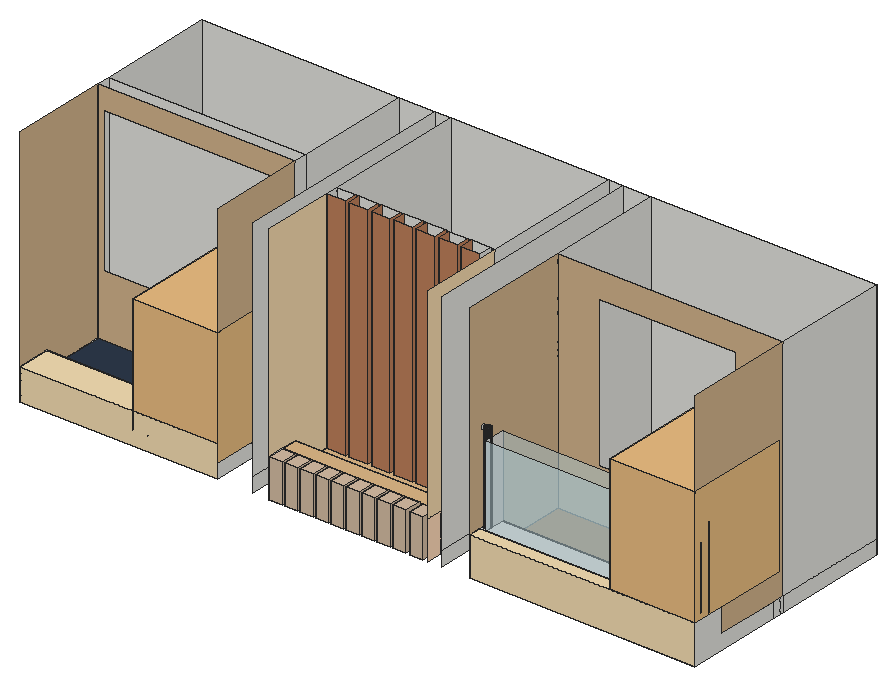
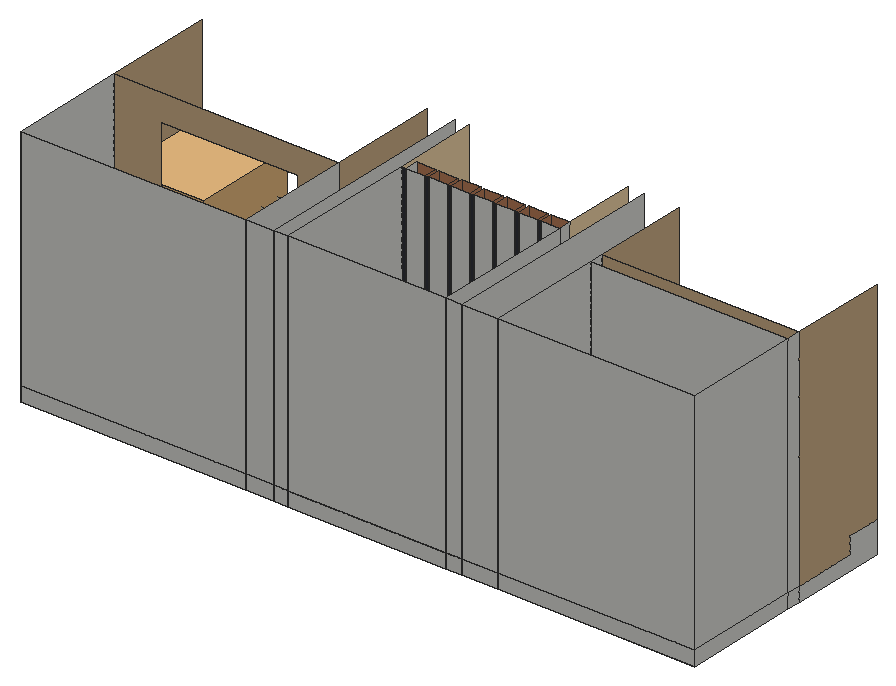
# SketchUp Ruby script. Lengths in inches.
U = 1.inch
M = Sketchup.active_model
def pt(a) = Geom::Point3d.new(a.map { |v| v * U })
def face(e, loops, mat)
  f = e.add_face(loops[0].map { |a| pt(a) })
  loops[1..].each { |l| e.add_face(l.map { |a| pt(a) }).erase! }
  f.material = f.back_material = mat if mat
  f
end
# faces: each face lists its corners as indices into pts; further lists are holes
def faces(e, pts, list, mat = nil) = list.each { |f| face(e, (f[0].is_a?(Array) ? f : [f]).map { |l| l.map { |i| pts[i] } }, mat) }
# xy, xz, yz: faces in a plane at the given z, y or x. An outline is a flat list of corners, or four numbers for a rectangle; further outlines are holes
def ring(l) = l.size == 4 ? [[l[0], l[1]], [l[2], l[1]], [l[2], l[3]], [l[0], l[3]]] : l.each_slice(2).to_a
def flat(e, list, mat, &to3) = list.each { |f| face(e, (f[0].is_a?(Array) ? f : [f]).map { |l| ring(l).map { |u, v| to3.(u, v) } }, mat) }
def xy(e, z, list, mat = nil) = flat(e, list, mat) { |x, y| [x, y, z] }
def xz(e, y, list, mat = nil) = flat(e, list, mat) { |x, z| [x, y, z] }
def yz(e, x, list, mat = nil) = flat(e, list, mat) { |y, z| [x, y, z] }
def lines(e, pts, list) = list.each { |a, b| e.add_line(pt(pts[a]), pt(pts[b])) }
# prism: a flat outline (further loops are holes) pulled along v
def prism(e, loops, v, mat = nil)
  f = face(e, loops, mat); d = Geom::Vector3d.new(v.map { |x| x * U })
  f.pushpull(f.normal.samedirection?(d) ? d.length : -d.length)
end
def box(e, o, s, mat = nil) = prism(e, [[o, [o[0] + s[0], o[1], o[2]], [o[0] + s[0], o[1] + s[1], o[2]], [o[0], o[1] + s[1], o[2]]]], [0, 0, s[2]], mat)
def at(x, y, z, deg = 0) = Geom::Transformation.translation(pt([x, y, z])) * Geom::Transformation.rotation(ORIGIN, Z_AXIS, deg.degrees)
def axes(o, x, y, z) = Geom::Transformation.new([*x, 0, *y, 0, *z, 0, *pt(o).to_a, 1])
def part(name) = M.definitions.add(name)
# library, detail: a bought-in or finely detailed component or shape, given as its bounding box
def library(name, o, s) = part(name).tap { |d| box(d.entities, o, s) }
def detail(e, o, s) = box(e.add_group.entities, o, s)
def put(e, d, t, mat = nil) = e.add_instance(d, t).tap { |i| i.material = mat if mat }
def group(e, t, mat = nil) = e.add_group.tap { |g| g.transformation = t; g.material = mat if mat }.entities
root = M.entities
M.materials.add("[0027_PeachPuff]").color = [255, 218, 185]
M.materials.add("[0034_Wheat]").color = [245, 222, 179]
M.materials.add("[0035_Tan]").color = [210, 180, 140]
M.materials.add("[0036_BurlyWood]1").color = [222, 184, 135]
M.materials.add("[Formica Beige]").color = [247, 219, 174]
M.materials.add("[Formica Laminate Dark]").color = [50, 53, 60]
M.materials.add("[Formica Laminate Light]").color = [213, 189, 164]
M.materials.add("[Leather Blue]").color = [45, 57, 74]
M.materials.add("[Translucent Glass Safety]").color = [204, 235, 244]
M.materials["[Translucent Glass Safety]"].alpha = 0.5
M.materials.add("[Wood Square Tile 02]").color = [160, 95, 34]
M.materials.add("[Wood Veneer 02]").color = [190, 128, 91]
c1 = library("chau cay",[-24.34,-109.24,0],[56.46,62.58,79.69])
xy(root,3076.3125,[[800.41,467.67,800.41,584.29,1272.8,584.29,1272.8,467.67,1233.94,467.67,1233.94,495.54,1224.82,495.54,1224.82,467.67,1185.96,467.67,1185.96,495.54,1176.83,495.54,1176.83,467.67,1137.97,467.67,1137.97,495.54,1128.4,495.54,1128.4,467.67,1089.53,467.67,1089.53,495.54,1080.21,495.54,1080.21,467.67,1041.35,467.67,1041.35,495.54,1032.02,495.54,1032.02,467.67,993.16,467.67,993.16,495.54,983.83,495.54,983.83,467.67,944.97,467.67,944.97,495.54,935.65,495.54,935.65,467.67,896.78,467.67,896.78,495.54,887.46,495.54,887.46,467.67,848.6,467.67,848.6,495.54,839.27,495.54,839.27,467.67],[800.41,467.67,839.27,495.54],[848.6,467.67,887.46,495.54],[896.78,467.67,935.65,495.54],[944.97,467.67,983.83,495.54],
  [993.16,467.67,1032.02,495.54],[1041.35,467.67,1080.21,495.54],[1089.53,467.67,1128.4,495.54],[1137.97,467.67,1176.83,495.54],[1185.96,467.67,1224.82,495.54],
  [1233.94,467.67,1272.8,495.54],[800.41,495.54,1272.8,584.29],[58.44,584.29,646.67,623.89],[646.67,584.29,752.97,623.89],[752.97,584.29,800.41,623.89],
  [800.41,584.29,1272.8,623.89],[1272.8,584.29,1313.62,623.89],[1313.62,584.29,1398.32,623.89],[1398.32,610.48,2069.85,623.89],[58.44,623.89,646.67,971.67],
  [646.67,623.89,752.97,971.67],[752.97,623.89,800.41,971.67],[800.41,623.89,1272.8,971.67],[1272.8,623.89,1313.62,971.67],[1313.62,623.89,1398.32,971.67],
  [1398.32,623.89,2069.85,971.67]])
xy(root,3076.3125,[[800.41,345.94,800.41,467.67,839.27,467.67,839.27,495.54,848.6,495.54,848.6,467.67,887.46,467.67,887.46,495.54,896.78,495.54,896.78,467.67,935.65,467.67,935.65,495.54,944.97,495.54,944.97,467.67,983.83,467.67,983.83,495.54,993.16,495.54,993.16,467.67,1032.02,467.67,1032.02,495.54,1041.35,495.54,1041.35,467.67,1080.21,467.67,1080.21,495.54,1089.53,495.54,1089.53,467.67,1128.4,467.67,1128.4,495.54,1137.97,495.54,1137.97,467.67,1176.83,467.67,1176.83,495.54,1185.96,495.54,1185.96,467.67,1224.82,467.67,1224.82,495.54,1233.94,495.54,1233.94,467.67,1272.8,467.67,1272.8,345.94]],"[0027_PeachPuff]")
xy(root,3076.3125,[[58.44,295.82,646.67,584.29],[1398.32,295.82,2069.85,584.29],[1398.32,584.29,2069.85,610.48]],"[0035_Tan]")
xy(root,3076.3125,[[800.41,295.82,840.47,345.94],[846.35,295.82,886.41,345.94],[892.28,295.82,932.35,345.94],[938.22,295.82,978.29,345.94],[984.16,295.82,1024.22,345.94],
  [1030.1,295.82,1070.16,345.94],[1076.03,295.82,1116.1,345.94],[1121.97,295.82,1162.04,345.94],[1167.91,295.82,1207.97,345.94],[1219.53,295.82,1259.6,345.94]],"[Formica Laminate Light]")
xy(root,3120,[[646.67,416.29,752.97,971.67],[752.97,416.29,800.41,971.67],[1272.8,416.29,1313.62,971.67],[1313.62,416.29,1398.32,971.67],[800.41,509.42,856.91,548.04],
  [867.28,509.42,923.79,548.04],[934.16,509.42,990.66,548.04],[1001.03,509.42,1057.54,548.04],[1067.91,509.42,1124.41,548.04],[1134.78,509.42,1191.29,548.04],
  [1201.66,509.42,1258.16,548.04],[800.41,548.04,1272.8,971.67],[58.44,584.29,646.67,623.89],[58.44,623.89,646.67,971.67],[1398.32,623.89,2069.85,971.67]])
xy(root,3120,[[800.41,393.82,1272.8,393.82,1272.8,548.04,1258.16,548.04,1258.16,509.42,1201.66,509.42,1201.66,548.04,1191.29,548.04,1191.29,509.42,1134.78,509.42,1134.78,548.04,1124.41,548.04,1124.41,509.42,1067.91,509.42,1067.91,548.04,1057.54,548.04,1057.54,509.42,1001.03,509.42,1001.03,548.04,990.66,548.04,990.66,509.42,934.16,509.42,934.16,548.04,923.79,548.04,923.79,509.42,867.28,509.42,867.28,548.04,856.91,548.04,856.91,509.42,800.41,509.42]],"[0036_BurlyWood]1")
xy(root,3120,[[58.44,393.82,646.67,584.29]],"[Leather Blue]")
xy(root,3120,[[1398.32,393.82,2069.85,623.89]],"[Wood Square Tile 02]")
xy(root,3171.25,[[58.44,295.82,646.67,393.82]],"[0034_Wheat]")
xy(root,3190.875,[[800.41,345.94,1272.8,393.82]],"[0036_BurlyWood]1")
xy(root,3190.875,[[800.41,295.82,840.47,345.94],[846.35,295.82,886.41,345.94],[892.28,295.82,932.35,345.94],[938.22,295.82,978.29,345.94],[984.16,295.82,1024.22,345.94],
  [1030.1,295.82,1070.16,345.94],[1076.03,295.82,1116.1,345.94],[1121.97,295.82,1162.04,345.94],[1167.91,295.82,1207.97,345.94],[1219.53,295.82,1259.6,345.94]],"[Formica Laminate Light]")
xy(root,3192.9375,[[[1398.32,332.12,1418.67,393.82],[1409.52,340.46,1407.29,340.76,1405.2,341.62,1403.42,342.99,1402.05,344.77,1401.1875,346.85,1400.89,349.09,1401.1875,351.32,1402.05,353.4,1403.42,355.1875,1405.2,356.56,1407.29,357.42,1409.52,357.71,1411.75,357.42,1413.83,356.56,1415.62,355.1875,1416.99,353.4,1417.85,351.32,1418.14,349.09,1417.85,346.85,1416.99,344.77,1415.62,342.99,1413.83,341.62,1411.75,340.76]],[1418.67,332.12,2047.84,393.82],[[2047.84,332.12,2069.85,393.82],[2057.02,340.46,2054.79,340.76,2052.7,341.62,2050.92,342.99,2049.55,344.77,2048.6875,346.85,2048.39,349.09,2048.6875,351.32,2049.55,353.4,2050.92,355.1875,2052.7,356.56,2054.79,357.42,2057.02,357.71,2059.25,357.42,2061.33,356.56,2063.12,355.1875,2064.49,353.4,2065.35,351.32,2065.64,349.09,2065.35,346.85,2064.49,344.77,2063.12,342.99,2061.33,341.62,2059.25,340.76]],[1409.52,340.46,1407.29,340.76,1405.2,341.62,1403.42,342.99,1402.05,344.77,1401.1875,346.85,1400.89,349.09,1401.1875,351.32,1402.05,353.4,1403.42,355.1875,1405.2,356.56,1407.29,357.42,1409.52,357.71,1411.75,357.42,1413.83,356.56,1415.62,355.1875,1416.99,353.4,1417.85,351.32,1418.14,349.09,1417.85,346.85,1416.99,344.77,1415.62,342.99,1413.83,341.62,1411.75,340.76],[2057.02,340.46,2054.79,340.76,2052.7,341.62,2050.92,342.99,2049.55,344.77,2048.6875,346.85,2048.39,349.09,2048.6875,351.32,2049.55,353.4,2050.92,355.1875,2052.7,356.56,2054.79,357.42,2057.02,357.71,2059.25,357.42,2061.33,356.56,2063.12,355.1875,2064.49,353.4,2065.35,351.32,2065.64,349.09,2065.35,346.85,2064.49,344.77,2063.12,342.99,2061.33,341.62,2059.25,340.76]])
xy(root,3192.9375,[[1398.32,295.82,2069.85,332.12]],"[0034_Wheat]")
xz(root,295.82,[[58.44,3076.3125,646.67,3171.25],[1398.32,3076.3125,2069.85,3192.9375]],"[0034_Wheat]")
xz(root,295.82,[[800.41,3076.3125,840.47,3190.875],[846.35,3076.3125,886.41,3190.875],[892.28,3076.3125,932.35,3190.875],[938.22,3076.3125,978.29,3190.875],[984.16,3076.3125,1024.22,3190.875],
  [1030.1,3076.3125,1070.16,3190.875],[1076.03,3076.3125,1116.1,3190.875],[1121.97,3076.3125,1162.04,3190.875],[1167.91,3076.3125,1207.97,3190.875],[1219.53,3076.3125,1259.6,3190.875]],"[Formica Laminate Light]")
xz(root,332.12,[[1418.67,3192.9375,2047.84,3433.875]],"[Translucent Glass Safety]")
xz(root,345.94,[[800.41,3076.3125,840.47,3190.875],[846.35,3076.3125,886.41,3190.875],[892.28,3076.3125,932.35,3190.875],[938.22,3076.3125,978.29,3190.875],[984.16,3076.3125,1024.22,3190.875],
  [1030.1,3076.3125,1070.16,3190.875],[1076.03,3076.3125,1116.1,3190.875],[1121.97,3076.3125,1162.04,3190.875],[1167.91,3076.3125,1207.97,3190.875],[1219.53,3076.3125,1259.6,3190.875]])
xz(root,345.94,[[840.47,3076.3125,846.35,3190.875],[886.41,3076.3125,892.28,3190.875],[932.35,3076.3125,938.22,3190.875],[978.29,3076.3125,984.16,3190.875],[1024.22,3076.3125,1030.1,3190.875],
  [1070.16,3076.3125,1076.03,3190.875],[1116.1,3076.3125,1121.97,3190.875],[1162.04,3076.3125,1167.91,3190.875],[1207.97,3076.3125,1219.53,3190.875],[1259.6,3076.3125,1272.8,3190.875]],"[Formica Laminate Dark]")
xz(root,393.82,[[1398.32,3120,2069.85,3192.9375]])
xz(root,393.82,[[58.44,3120,646.67,3171.25]],"[0034_Wheat]")
xz(root,393.82,[[800.41,3120,1272.8,3190.875]],"[0036_BurlyWood]1")
xz(root,393.82,[[1418.67,3192.9375,2047.84,3433.875]],"[Translucent Glass Safety]")
xz(root,509.42,[[800.41,3120,856.91,3798.8125],[867.28,3120,923.79,3798.8125],[934.16,3120,990.66,3798.8125],[1001.03,3120,1057.54,3798.8125],[1067.91,3120,1124.41,3798.8125],
  [1134.78,3120,1191.29,3798.8125],[1201.66,3120,1258.16,3798.8125]],"[Wood Veneer 02]")
xz(root,548.04,[[800.41,3120,856.91,3798.8125],[867.28,3120,923.79,3798.8125],[934.16,3120,990.66,3798.8125],[1001.03,3120,1057.54,3798.8125],[1067.91,3120,1124.41,3798.8125],
  [1134.78,3120,1191.29,3798.8125],[1201.66,3120,1258.16,3798.8125]])
xz(root,548.04,[[856.91,3120,867.28,3798.8125],[923.79,3120,934.16,3798.8125],[990.66,3120,1001.03,3798.8125],[1057.54,3120,1067.91,3798.8125],[1124.41,3120,1134.78,3798.8125],
  [1191.29,3120,1201.66,3798.8125],[1258.16,3120,1272.8,3798.8125]],"[Formica Laminate Dark]")
xz(root,584.29,[[[58.44,3120,646.67,3798.8125],[76.9,3305.37,630.15,3735.8]]],"[0035_Tan]")
xz(root,623.89,[[58.44,3120,646.67,3798.8125]])
xz(root,623.89,[[[1398.32,3120,2069.85,3798.8125],[1520.9,3276.35,1928.53,3721.73]]],"[0035_Tan]")
xz(root,971.67,[[58.44,3076.3125,646.67,3120],[646.67,3076.3125,752.97,3120],[752.97,3076.3125,800.41,3120],[800.41,3076.3125,1272.8,3120],[1272.8,3076.3125,1313.62,3120],
  [1313.62,3076.3125,1398.32,3120],[1398.32,3076.3125,2069.85,3120],[58.44,3120,646.67,3798.8125],[646.67,3120,752.97,3798.8125],[752.97,3120,800.41,3798.8125],
  [800.41,3120,1272.8,3798.8125],[1272.8,3120,1313.62,3798.8125],[1313.62,3120,1398.32,3798.8125],[1398.32,3120,2069.85,3798.8125]])
yz(root,58.44,[[295.82,3076.3125,295.82,3171.25,393.82,3171.25,393.82,3120,584.29,3120,584.29,3076.3125],[584.29,3076.3125,623.89,3120],[623.89,3076.3125,971.67,3120],[584.29,3120,623.89,3798.8125],[623.89,3120,971.67,3798.8125]])
yz(root,58.44,[[393.82,3120,584.29,3120,584.29,3798.8125,295.82,3798.8125,295.82,3171.25,393.82,3171.25]],"[0035_Tan]")
yz(root,646.67,[[295.82,3076.3125,971.67,3120],[295.82,3120,393.82,3171.25],[584.29,3120,623.89,3798.8125],[623.89,3120,971.67,3798.8125]])
yz(root,646.67,[[393.82,3120,393.82,3171.25,295.82,3171.25,295.82,3798.8125,584.29,3798.8125,584.29,3120]],"[0035_Tan]")
yz(root,752.97,[[295.82,3076.3125,971.67,3120],[295.82,3120,971.67,3798.8125]])
yz(root,800.41,[[295.82,3076.3125,345.94,3120],[345.94,3076.3125,971.67,3120],[295.82,3120,345.94,3190.875],[345.94,3120,393.82,3190.875],[509.42,3120,548.04,3798.8125],
  [548.04,3120,971.67,3798.8125]])
yz(root,800.41,[[393.82,3120,509.42,3120,509.42,3798.8125,295.82,3798.8125,295.82,3190.875,393.82,3190.875]],"[Formica Beige]")
yz(root,840.47,[[295.82,3076.3125,345.94,3190.875]],"[Formica Laminate Light]")
yz(root,846.35,[[295.82,3076.3125,345.94,3120],[295.82,3120,345.94,3190.875]],"[Formica Laminate Light]")
yz(root,856.91,[[509.42,3120,548.04,3798.8125]],"[Wood Veneer 02]")
yz(root,867.28,[[509.42,3120,548.04,3798.8125]],"[Wood Veneer 02]")
yz(root,886.41,[[295.82,3076.3125,345.94,3190.875]],"[Formica Laminate Light]")
yz(root,892.28,[[295.82,3076.3125,345.94,3120],[295.82,3120,345.94,3190.875]],"[Formica Laminate Light]")
yz(root,923.79,[[509.42,3120,548.04,3798.8125]],"[Wood Veneer 02]")
yz(root,932.35,[[295.82,3076.3125,345.94,3190.875]],"[Formica Laminate Light]")
yz(root,934.16,[[509.42,3120,548.04,3798.8125]],"[Wood Veneer 02]")
yz(root,938.22,[[295.82,3076.3125,345.94,3120],[295.82,3120,345.94,3190.875]],"[Formica Laminate Light]")
yz(root,978.29,[[295.82,3076.3125,345.94,3190.875]],"[Formica Laminate Light]")
yz(root,984.16,[[295.82,3076.3125,345.94,3120],[295.82,3120,345.94,3190.875]],"[Formica Laminate Light]")
yz(root,990.66,[[509.42,3120,548.04,3798.8125]],"[Wood Veneer 02]")
yz(root,1001.03,[[509.42,3120,548.04,3798.8125]],"[Wood Veneer 02]")
yz(root,1024.22,[[295.82,3076.3125,345.94,3190.875]],"[Formica Laminate Light]")
yz(root,1030.1,[[295.82,3076.3125,345.94,3120],[295.82,3120,345.94,3190.875]],"[Formica Laminate Light]")
yz(root,1057.54,[[509.42,3120,548.04,3798.8125]],"[Wood Veneer 02]")
yz(root,1067.91,[[509.42,3120,548.04,3798.8125]],"[Wood Veneer 02]")
yz(root,1070.16,[[295.82,3076.3125,345.94,3190.875]],"[Formica Laminate Light]")
yz(root,1076.03,[[295.82,3076.3125,345.94,3120],[295.82,3120,345.94,3190.875]],"[Formica Laminate Light]")
yz(root,1116.1,[[295.82,3076.3125,345.94,3190.875]],"[Formica Laminate Light]")
yz(root,1121.97,[[295.82,3076.3125,345.94,3120],[295.82,3120,345.94,3190.875]],"[Formica Laminate Light]")
yz(root,1124.41,[[509.42,3120,548.04,3798.8125]],"[Wood Veneer 02]")
yz(root,1134.78,[[509.42,3120,548.04,3798.8125]],"[Wood Veneer 02]")
yz(root,1162.04,[[295.82,3076.3125,345.94,3190.875]],"[Formica Laminate Light]")
yz(root,1167.91,[[295.82,3076.3125,345.94,3120],[295.82,3120,345.94,3190.875]],"[Formica Laminate Light]")
yz(root,1191.29,[[509.42,3120,548.04,3798.8125]],"[Wood Veneer 02]")
yz(root,1201.66,[[509.42,3120,548.04,3798.8125]],"[Wood Veneer 02]")
yz(root,1207.97,[[295.82,3076.3125,345.94,3190.875]],"[Formica Laminate Light]")
yz(root,1219.53,[[295.82,3076.3125,345.94,3120],[295.82,3120,345.94,3190.875]],"[Formica Laminate Light]")
yz(root,1258.16,[[509.42,3120,548.04,3798.8125]])
yz(root,1259.6,[[295.82,3076.3125,345.94,3190.875]],"[Formica Laminate Light]")
yz(root,1272.8,[[345.94,3076.3125,971.67,3120],[345.94,3120,393.82,3190.875],[548.04,3120,971.67,3798.8125]])
yz(root,1272.8,[[295.82,3076.3125,345.94,3190.875]],"[0027_PeachPuff]")
yz(root,1272.8,[[393.82,3120,393.82,3190.875,295.82,3190.875,295.82,3798.8125,548.04,3798.8125,548.04,3120]],"[Formica Beige]")
yz(root,1313.62,[[295.82,3076.3125,971.67,3120],[295.82,3120,971.67,3798.8125]])
yz(root,1398.32,[[295.82,3076.3125,971.67,3120],[295.82,3120,393.82,3192.9375],[623.89,3120,971.67,3798.8125]])
yz(root,1398.32,[[[393.82,3120,623.89,3120,623.89,3798.8125,295.82,3798.8125,295.82,3192.9375,393.82,3192.9375],[344.51,3450.8125,342.28,3451.11,340.2,3451.97,338.41,3453.34,337.04,3455.125,336.18,3457.21,335.89,3459.4375,336.18,3461.67,337.04,3463.75,338.41,3465.54,340.2,3466.91,342.28,3467.77,344.51,3468.0625,346.74,3467.77,348.82,3466.91,350.61,3465.54,351.98,3463.75,352.84,3461.67,353.14,3459.4375,352.84,3457.21,351.98,3455.125,350.61,3453.34,348.82,3451.97,346.74,3451.11]]],"[0035_Tan]")
yz(root,1418.67,[[332.12,3192.9375,393.82,3433.875]])
yz(root,2047.84,[[332.12,3192.9375,393.82,3433.875]])
yz(root,2069.85,[[295.82,3076.3125,584.29,3076.3125,584.29,3120,393.82,3120,393.82,3192.9375,295.82,3192.9375],[584.29,3076.3125,610.48,3120],[610.48,3076.3125,623.89,3120],[623.89,3076.3125,971.67,3120],[623.89,3120,971.67,3798.8125]])
yz(root,2069.85,[[[393.82,3120,393.82,3192.9375,295.82,3192.9375,295.82,3798.8125,623.89,3798.8125,623.89,3120],[344.51,3450.8125,346.74,3451.11,348.82,3451.97,350.61,3453.34,351.98,3455.125,352.84,3457.21,353.14,3459.4375,352.84,3461.67,351.98,3463.75,350.61,3465.54,348.82,3466.91,346.74,3467.77,344.51,3468.0625,342.28,3467.77,340.2,3466.91,338.41,3465.54,337.04,3463.75,336.18,3461.67,335.89,3459.4375,336.18,3457.21,337.04,3455.125,338.41,3453.34,340.2,3451.97,342.28,3451.11]]],"[0035_Tan]")
p = [[1407.29,340.76,3192.9375],[1409.52,340.46,3192.9375],[1409.52,340.46,3461.67],[1407.29,340.76,3461.67],[1411.75,340.76,3192.9375],[1411.75,340.76,3461.67],
  [2054.79,340.76,3192.9375],[2057.02,340.46,3192.9375],[2057.02,340.46,3459.4375],[2054.79,340.76,3459.4375],[2059.25,340.76,3192.9375],[2059.25,340.76,3459.4375],
  [1405.2,341.62,3192.9375],[1405.2,341.62,3461.67],[1413.83,341.62,3192.9375],[1413.83,341.62,3461.67],[2052.7,341.62,3192.9375],[2052.7,341.62,3459.4375],
  [2061.33,341.62,3192.9375],[2061.33,341.62,3459.4375],[1403.42,342.99,3192.9375],[1403.42,342.99,3461.67],[1415.62,342.99,3192.9375],[1415.62,342.99,3461.67],
  [2050.92,342.99,3192.9375],[2050.92,342.99,3459.4375],[2063.12,342.99,3192.9375],[2063.12,342.99,3459.4375],[1402.05,344.77,3192.9375],[1402.05,344.77,3461.67],
  [1416.99,344.77,3192.9375],[1416.99,344.77,3461.67],[2049.55,344.77,3192.9375],[2049.55,344.77,3459.4375],[2064.49,344.77,3192.9375],[2064.49,344.77,3459.4375],
  [1401.1875,346.85,3192.9375],[1401.1875,346.85,3461.67],[1417.85,346.85,3192.9375],[1417.85,346.85,3461.67],[2048.6875,346.85,3192.9375],[2048.6875,346.85,3459.4375],
  [2065.35,346.85,3192.9375],[2065.35,346.85,3459.4375],[1400.89,349.09,3192.9375],[1400.89,349.09,3461.67],[1418.14,349.09,3192.9375],[1418.14,349.09,3461.67],
  [2048.39,349.09,3192.9375],[2048.39,349.09,3459.4375],[2065.64,349.09,3192.9375],[2065.64,349.09,3459.4375],[1401.1875,351.32,3192.9375],[1401.1875,351.32,3461.67],
  [1417.85,351.32,3192.9375],[1417.85,351.32,3461.67],[2048.6875,351.32,3192.9375],[2048.6875,351.32,3459.4375],[2065.35,351.32,3192.9375],[2065.35,351.32,3459.4375],
  [1402.05,353.4,3192.9375],[1401.82,352.84,3461.67],[1402.05,353.4,3461.67],[1416.99,353.4,3192.9375],[1416.99,353.4,3461.67],[1417.22,352.84,3461.67],
  [2049.55,353.4,3192.9375],[2049.4375,353.14,3459.4375],[2049.55,353.4,3459.4375],[2064.49,353.4,3192.9375],[2064.49,353.4,3459.4375],[2064.6,353.14,3459.4375],
  [1403.42,355.1875,3192.9375],[1403.42,355.1875,3461.67],[1415.62,355.1875,3192.9375],[1415.62,355.1875,3461.67],[2050.92,355.1875,3192.9375],[2050.92,355.1875,3459.4375],
  [2063.12,355.1875,3192.9375],[2063.12,355.1875,3459.4375],[1405.2,356.56,3192.9375],[1405.2,356.56,3461.67],[1413.83,356.56,3192.9375],[1413.83,356.56,3461.67],
  [2052.7,356.56,3192.9375],[2052.7,356.56,3459.4375],[2061.33,356.56,3192.9375],[2061.33,356.56,3459.4375],[1407.29,357.42,3192.9375],[1407.29,357.42,3461.67],
  [1411.75,357.42,3192.9375],[1411.75,357.42,3461.67],[2054.79,357.42,3192.9375],[2054.79,357.42,3459.4375],[2059.25,357.42,3192.9375],[2059.25,357.42,3459.4375],
  [1409.52,357.71,3192.9375],[1409.52,357.71,3461.67],[2057.02,357.71,3192.9375],[2057.02,357.71,3459.4375]]
faces(root,p,[[0,1,2,3],[1,4,5,2],[6,7,8,9],[7,10,11,8],[12,0,3,13],[4,14,15,5],[16,6,9,17],[10,18,19,11],
  [20,12,13,21],[14,22,23,15],[24,16,17,25],[18,26,27,19],[28,20,21,29],[22,30,31,23],[32,24,25,33],[26,34,35,27],
  [36,28,29,37],[30,38,39,31],[40,32,33,41],[34,42,43,35],[44,36,37,45],[38,46,47,39],[48,40,41,49],[42,50,51,43],
  [52,44,45,53],[46,54,55,47],[56,48,49,57],[50,58,59,51],[60,52,53,61,62],[54,63,64,65,55],[66,56,57,67,68],[58,69,70,71,59],
  [72,60,62,73],[63,74,75,64],[76,66,68,77],[69,78,79,70],[80,72,73,81],[74,82,83,75],[84,76,77,85],[78,86,87,79],
  [88,80,81,89],[82,90,91,83],[92,84,85,93],[86,94,95,87],[96,88,89,97],[90,96,97,91],[98,92,93,99],[94,98,99,95]],"[Formica Laminate Dark]")
put(root,c1,axes([502.14,64.16,3120],[4.5,0,0],[0,-4.9651,0],[0,0,4.37432]))
put(root,c1,axes([1925.3125,64.16,3192.9375],[4.5,0,0],[0,-4.9651,0],[0,0,4.37432]))
